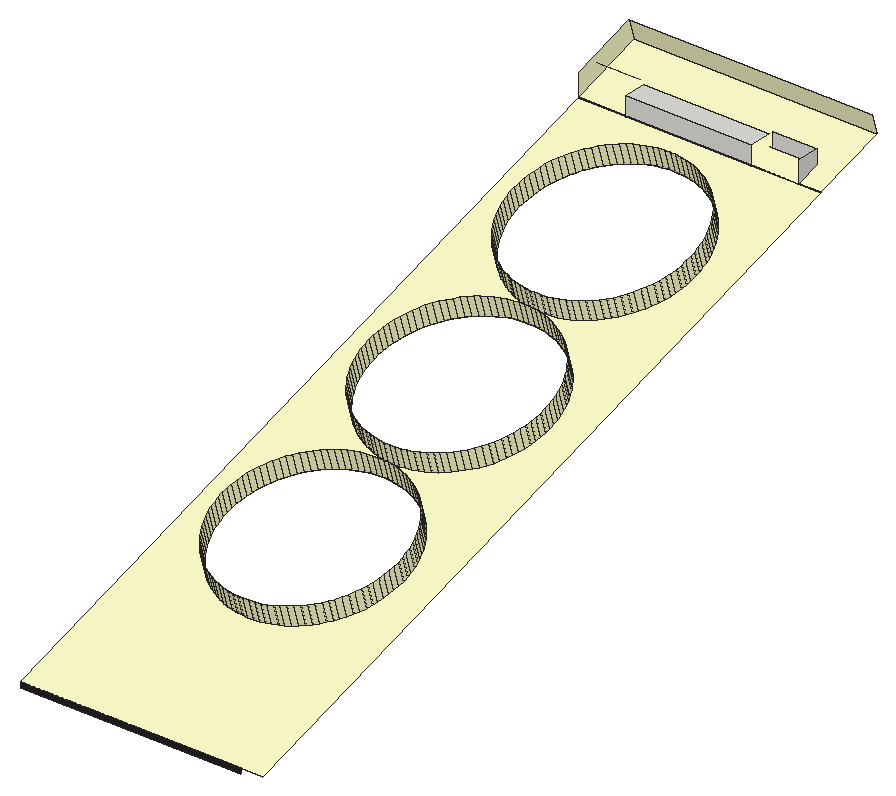
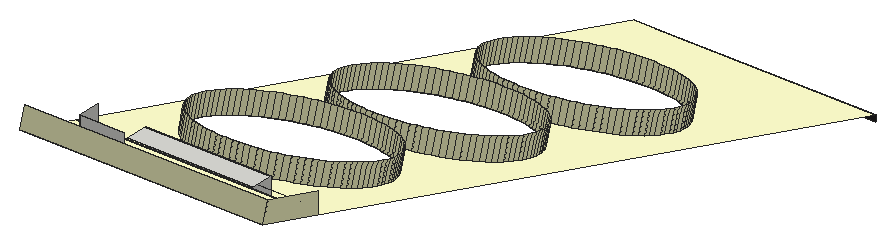
# SketchUp Ruby script. Lengths in inches.
U = 1.inch
M = Sketchup.active_model
def pt(a) = Geom::Point3d.new(a.map { |v| v * U })
def face(e, loops, mat)
  f = e.add_face(loops[0].map { |a| pt(a) })
  loops[1..].each { |l| e.add_face(l.map { |a| pt(a) }).erase! }
  f.material = f.back_material = mat if mat
  f
end
# faces: each face lists its corners as indices into pts; further lists are holes
def faces(e, pts, list, mat = nil) = list.each { |f| face(e, (f[0].is_a?(Array) ? f : [f]).map { |l| l.map { |i| pts[i] } }, mat) }
# xy, xz, yz: faces in a plane at the given z, y or x. An outline is a flat list of corners, or four numbers for a rectangle; further outlines are holes
def ring(l) = l.size == 4 ? [[l[0], l[1]], [l[2], l[1]], [l[2], l[3]], [l[0], l[3]]] : l.each_slice(2).to_a
def flat(e, list, mat, &to3) = list.each { |f| face(e, (f[0].is_a?(Array) ? f : [f]).map { |l| ring(l).map { |u, v| to3.(u, v) } }, mat) }
def xy(e, z, list, mat = nil) = flat(e, list, mat) { |x, y| [x, y, z] }
def xz(e, y, list, mat = nil) = flat(e, list, mat) { |x, z| [x, y, z] }
def yz(e, x, list, mat = nil) = flat(e, list, mat) { |y, z| [x, y, z] }
def lines(e, pts, list) = list.each { |a, b| e.add_line(pt(pts[a]), pt(pts[b])) }
# prism: a flat outline (further loops are holes) pulled along v
def prism(e, loops, v, mat = nil)
  f = face(e, loops, mat); d = Geom::Vector3d.new(v.map { |x| x * U })
  f.pushpull(f.normal.samedirection?(d) ? d.length : -d.length)
end
def box(e, o, s, mat = nil) = prism(e, [[o, [o[0] + s[0], o[1], o[2]], [o[0] + s[0], o[1] + s[1], o[2]], [o[0], o[1] + s[1], o[2]]]], [0, 0, s[2]], mat)
def at(x, y, z, deg = 0) = Geom::Transformation.translation(pt([x, y, z])) * Geom::Transformation.rotation(ORIGIN, Z_AXIS, deg.degrees)
def axes(o, x, y, z) = Geom::Transformation.new([*x, 0, *y, 0, *z, 0, *pt(o).to_a, 1])
def part(name) = M.definitions.add(name)
# library, detail: a bought-in or finely detailed component or shape, given as its bounding box
def library(name, o, s) = part(name).tap { |d| box(d.entities, o, s) }
def detail(e, o, s) = box(e.add_group.entities, o, s)
def put(e, d, t, mat = nil) = e.add_instance(d, t).tap { |i| i.material = mat if mat }
def group(e, t, mat = nil) = e.add_group.tap { |g| g.transformation = t; g.material = mat if mat }.entities
root = M.entities
M.materials.add("E01_Mint_Frost").color = [255, 255, 204]
M.materials.add("Marble_07_1K").color = [36, 34, 36]
xy(root,503,[[276.5,247,310.5,253]])
xz(root,57,[[263.5,437.47,323.5,439.04]],"Marble_07_1K")
xz(root,247,[[263.5,498,276.5,498.15],[276.5,498,310.5,498.15],[310.5,498,323.5,498.15],[323.5,498,329.5,498.15],[276.5,498.15,310.5,503]])
xz(root,253,[[311.5,500.01,323.5,504]])
yz(root,263.5,[[247,498.15,247,504,264.19,509.34,265.85,504,253,500.01]],"E01_Mint_Frost")
yz(root,323.5,[[247,498.15,253,500.01,253,504,247,504]])
p = [[323.5,57,439.04],[263.5,57,439.04],[263.5,247,498],[276.5,247,498],[310.5,247,498],[317.5,247,498],
  [323.5,247,498],[329.5,247,498],[329.5,57,439.04],[273.25,171.72,474.64],[272.93,170.32,474.2],[272.6875,168.89,473.76],
  [272.55,167.46,473.32],[272.5,166.02,472.87],[272.55,164.58,472.42],[272.6875,163.15,471.98],[272.93,161.73,471.54],[273.25,160.32,471.1],
  [273.67,158.9375,470.67],[274.19,157.58,470.25],[274.78,156.26,469.84],[275.47,154.98,469.44],[276.24,153.74,469.06],[277.08,152.55,468.6875],
  [278.01,151.41,468.33],[279,150.33,468],[280.07,149.3125,467.68],[281.2,148.36,467.39],[282.39,147.48,467.11],[283.64,146.67,466.86],
  [284.9375,145.93,466.64],[286.28,145.28,466.43],[287.67,144.71,466.25],[289.08,144.22,466.1],[290.53,143.82,465.98],[292,143.51,465.88],
  [293.49,143.28,465.8125],[294.99,143.14,465.77],[296.5,143.1,465.76],[298.01,143.14,465.77],[299.51,143.28,465.8125],[301,143.51,465.88],
  [302.47,143.82,465.98],[303.92,144.22,466.1],[305.33,144.71,466.25],[306.72,145.28,466.43],[308.0625,145.93,466.64],[309.36,146.67,466.86],
  [310.61,147.48,467.11],[311.8,148.36,467.39],[312.93,149.3125,467.68],[314,150.33,468],[314.99,151.41,468.33],[315.92,152.55,468.6875],
  [316.76,153.74,469.06],[317.53,154.98,469.44],[318.22,156.26,469.84],[318.81,157.58,470.25],[319.33,158.9375,470.67],[319.75,160.32,471.1],
  [320.07,161.73,471.54],[320.3125,163.15,471.98],[320.45,164.58,472.42],[320.5,166.02,472.87],[320.45,167.46,473.32],[320.3125,168.89,473.76],
  [320.07,170.32,474.2],[319.75,171.72,474.64],[319.33,173.1,475.07],[318.81,174.46,475.49],[318.22,175.78,475.9],[317.53,177.0625,476.3],
  [316.76,178.3,476.68],[315.92,179.49,477.05],[314.99,180.63,477.4],[314,181.71,477.74],[312.93,182.73,478.05],[311.8,183.68,478.35],
  [310.61,184.57,478.625],[309.36,185.375,478.875],[308.0625,186.11,479.1],[306.72,186.76,479.31],[305.33,187.33,479.48],[303.92,187.82,479.63],
  [302.47,188.22,479.76],[301,188.54,479.86],[299.51,188.76,479.93],[298.01,188.9,479.97],[296.5,188.94,479.98],[294.99,188.9,479.97],
  [293.49,188.76,479.93],[292,188.54,479.86],[290.53,188.22,479.76],[289.08,187.82,479.63],[287.67,187.33,479.48],[286.28,186.76,479.31],
  [284.9375,186.11,479.1],[283.64,185.375,478.875],[282.39,184.57,478.625],[281.2,183.68,478.35],[280.07,182.73,478.05],[279,181.71,477.74],
  [278.01,180.63,477.4],[277.08,179.49,477.05],[276.24,178.3,476.68],[275.47,177.0625,476.3],[274.78,175.78,475.9],[274.19,174.46,475.49],
  [273.67,173.1,475.07],[272.6875,218.44,489.14],[272.55,217.01,488.69],[272.5,215.57,488.25],[272.55,214.13,487.8],[272.6875,212.7,487.35],
  [272.93,211.28,486.91],[273.25,209.87,486.48],[273.67,208.49,486.05],[274.19,207.13,485.63],[274.78,205.8125,485.22],[275.47,204.53,484.82],
  [276.24,203.29,484.43],[277.08,202.1,484.06],[278.01,200.96,483.71],[279,199.88,483.375],[280.07,198.86,483.0625],[281.2,197.91,482.77],
  [282.39,197.03,482.49],[283.64,196.22,482.24],[284.9375,195.48,482.01],[286.28,194.83,481.81],[287.67,194.26,481.63],[289.08,193.77,481.48],
  [290.53,193.37,481.36],[292,193.06,481.26],[293.49,192.83,481.1875],[294.99,192.69,481.15],[296.5,192.65,481.13],[298.01,192.69,481.15],
  [299.51,192.83,481.1875],[301,193.06,481.26],[302.47,193.37,481.36],[303.92,193.77,481.48],[305.33,194.26,481.63],[306.72,194.83,481.81],
  [308.0625,195.48,482.01],[309.36,196.22,482.24],[310.61,197.03,482.49],[311.8,197.91,482.77],[312.93,198.86,483.0625],[314,199.88,483.375],
  [314.99,200.96,483.71],[315.92,202.1,484.06],[316.76,203.29,484.43],[317.53,204.53,484.82],[318.22,205.8125,485.22],[318.81,207.13,485.63],
  [319.33,208.49,486.05],[319.75,209.87,486.48],[320.07,211.28,486.91],[320.3125,212.7,487.35],[320.45,214.13,487.8],[320.5,215.57,488.25],
  [320.45,217.01,488.69],[320.3125,218.44,489.14],[320.07,219.87,489.58],[319.75,221.27,490.02],[319.33,222.65,490.44],[318.81,224.01,490.86],
  [318.22,225.33,491.27],[317.53,226.61,491.67],[316.76,227.85,492.06],[315.92,229.04,492.43],[314.99,230.18,492.78],[314,231.26,493.12],
  [312.93,232.28,493.43],[311.8,233.23,493.73],[310.61,234.11,494],[309.36,234.92,494.25],[308.0625,235.66,494.48],[306.72,236.3125,494.68],
  [305.33,236.88,494.86],[303.92,237.37,495.01],[302.47,237.77,495.14],[301,238.09,495.23],[299.51,238.3125,495.3],[298.01,238.45,495.35],
  [296.5,238.49,495.36],[294.99,238.45,495.35],[293.49,238.3125,495.3],[292,238.09,495.23],[290.53,237.77,495.14],[289.08,237.37,495.01],
  [287.67,236.88,494.86],[286.28,236.3125,494.68],[284.9375,235.66,494.48],[283.64,234.92,494.25],[282.39,234.11,494],[281.2,233.23,493.73],
  [280.07,232.28,493.43],[279,231.26,493.12],[278.01,230.18,492.78],[277.08,229.04,492.43],[276.24,227.85,492.06],[275.47,226.61,491.67],
  [274.78,225.33,491.27],[274.19,224.01,490.86],[273.67,222.65,490.44],[273.25,221.27,490.02],[272.93,219.87,489.58],[274.19,124.58,460.01],
  [273.67,123.23,459.59],[273.25,121.84,459.16],[272.93,120.4375,458.72],[272.6875,119.02,458.28],[272.55,117.58,457.84],[272.5,116.14,457.39],
  [272.55,114.7,456.94],[272.6875,113.27,456.5],[272.93,111.85,456.06],[273.25,110.44,455.62],[273.67,109.06,455.19],[274.19,107.71,454.77],
  [274.78,106.38,454.36],[275.47,105.1,453.96],[276.24,103.86,453.58],[277.08,102.67,453.21],[278.01,101.53,452.86],[279,100.45,452.52],
  [280.07,99.43,452.2],[281.2,98.48,451.91],[282.39,97.6,451.63],[283.64,96.79,451.38],[284.9375,96.06,451.16],[286.28,95.4,450.95],
  [287.67,94.83,450.78],[289.08,94.34,450.625],[290.53,93.94,450.5],[292,93.63,450.4],[293.49,93.4,450.33],[294.99,93.27,450.29],
  [296.5,93.22,450.28],[298.01,93.27,450.29],[299.51,93.4,450.33],[301,93.63,450.4],[302.47,93.94,450.5],[303.92,94.34,450.625],
  [305.33,94.83,450.78],[306.72,95.4,450.95],[308.0625,96.06,451.16],[309.36,96.79,451.38],[310.61,97.6,451.63],[311.8,98.48,451.91],
  [312.93,99.43,452.2],[314,100.45,452.52],[314.99,101.53,452.86],[315.92,102.67,453.21],[316.76,103.86,453.58],[317.53,105.1,453.96],
  [318.22,106.38,454.36],[318.81,107.71,454.77],[319.33,109.06,455.19],[319.75,110.44,455.62],[320.07,111.85,456.06],[320.3125,113.27,456.5],
  [320.45,114.7,456.94],[320.5,116.14,457.39],[320.45,117.58,457.84],[320.3125,119.02,458.28],[320.07,120.4375,458.72],[319.75,121.84,459.16],
  [319.33,123.23,459.59],[318.81,124.58,460.01],[318.22,125.9,460.42],[317.53,127.1875,460.82],[316.76,128.43,461.2],[315.92,129.62,461.57],
  [314.99,130.75,461.92],[314,131.83,462.26],[312.93,132.85,462.57],[311.8,133.8,462.87],[310.61,134.6875,463.14],[309.36,135.5,463.4],
  [308.0625,136.23,463.625],[306.72,136.88,463.83],[305.33,137.46,464],[303.92,137.94,464.15],[302.47,138.34,464.28],[301,138.66,464.375],
  [299.51,138.88,464.45],[298.01,139.02,464.49],[296.5,139.06,464.5],[294.99,139.02,464.49],[293.49,138.88,464.45],[292,138.66,464.375],
  [290.53,138.34,464.28],[289.08,137.94,464.15],[287.67,137.46,464],[286.28,136.88,463.83],[284.9375,136.23,463.625],[283.64,135.5,463.4],
  [282.39,134.6875,463.14],[281.2,133.8,462.87],[280.07,132.85,462.57],[279,131.83,462.26],[278.01,130.75,461.92],[277.08,129.62,461.57],
  [276.24,128.43,461.2],[275.47,127.1875,460.82],[274.78,125.9,460.42],[294.99,91.57,455.76],[295.01,91.57,455.76],[296.5,91.52,455.75],
  [297.99,91.57,455.76],[298.01,91.57,455.76],[293.49,91.7,455.8],[299.51,91.7,455.8],[292,91.93,455.875],[301,91.93,455.875],
  [290.53,92.24,455.97],[302.47,92.24,455.97],[289.08,92.65,456.1],[303.92,92.65,456.1],[287.67,93.13,456.25],[305.33,93.13,456.25],
  [286.28,93.7,456.43],[306.72,93.7,456.43],[284.9375,94.36,456.63],[308.0625,94.36,456.63],[283.64,95.09,456.86],[309.36,95.09,456.86],
  [282.39,95.9,457.11],[310.61,95.9,457.11],[281.2,96.78,457.38],[311.8,96.78,457.38],[280.07,97.74,457.68],[312.93,97.74,457.68],
  [279,98.75,457.99],[314,98.75,457.99],[278.01,99.83,458.33],[314.99,99.83,458.33],[277.08,100.97,458.68],[315.92,100.97,458.68],
  [276.24,102.16,459.05],[316.76,102.16,459.05],[275.47,103.4,459.44],[317.53,103.4,459.44],[274.78,104.69,459.83],[318.22,104.69,459.83],
  [274.19,106.01,460.24],[318.81,106.01,460.24],[273.67,107.36,460.66],[319.33,107.36,460.66],[273.25,108.74,461.09],[319.75,108.74,461.09],
  [272.93,110.15,461.53],[320.07,110.15,461.53],[272.6875,111.57,461.97],[320.3125,111.57,461.97],[272.55,113.01,462.42],[320.45,113.01,462.42],
  [272.5,114.44,462.86],[320.5,114.44,462.86],[272.55,115.88,463.31],[320.45,115.88,463.31],[272.6875,117.32,463.75],[320.3125,117.32,463.75],
  [272.93,118.74,464.2],[320.07,118.74,464.2],[273.25,120.15,464.63],[319.75,120.15,464.63],[273.67,121.53,465.06],[319.33,121.53,465.06],
  [274.19,122.88,465.48],[318.81,122.88,465.48],[274.78,124.2,465.89],[318.22,124.2,465.89],[275.47,125.49,466.29],[317.53,125.49,466.29],
  [276.24,126.73,466.67],[316.76,126.73,466.67],[277.08,127.92,467.04],[315.92,127.92,467.04],[278.01,129.06,467.4],[314.99,129.06,467.4],
  [279,130.14,467.73],[314,130.14,467.73],[280.07,131.15,468.05],[312.93,131.15,468.05],[281.2,132.11,468.34],[311.8,132.11,468.34],
  [282.39,132.99,468.62],[310.61,132.99,468.62],[283.64,133.8,468.87],[309.36,133.8,468.87],[284.9375,134.53,469.1],[308.0625,134.53,469.1],
  [286.28,135.18,469.3],[306.72,135.18,469.3],[287.67,135.76,469.48],[305.33,135.76,469.48],[289.08,136.24,469.63],[303.92,136.24,469.63],
  [290.53,136.65,469.75],[302.47,136.65,469.75],[292,136.96,469.85],[301,136.96,469.85],[293.49,137.1875,469.92],[299.51,137.1875,469.92],
  [294.99,137.32,469.96],[298.01,137.32,469.96],[296.5,137.37,469.98],[293.49,141.58,471.28],[294.99,141.45,471.24],[296.5,141.4,471.23],
  [298.01,141.45,471.24],[299.51,141.58,471.28],[292,141.81,471.35],[301,141.81,471.35],[290.53,142.12,471.45],[302.47,142.12,471.45],
  [289.08,142.52,471.58],[303.92,142.52,471.58],[287.67,143.01,471.73],[305.33,143.01,471.73],[286.28,143.58,471.91],[306.72,143.58,471.91],
  [284.9375,144.24,472.11],[308.0625,144.24,472.11],[283.64,144.97,472.34],[309.36,144.97,472.34],[282.39,145.78,472.59],[310.61,145.78,472.59],
  [281.2,146.66,472.86],[311.8,146.66,472.86],[280.07,147.61,473.16],[312.93,147.61,473.16],[279,148.63,473.47],[314,148.63,473.47],
  [278.01,149.71,473.81],[314.99,149.71,473.81],[277.08,150.85,474.16],[315.92,150.85,474.16],[276.24,152.04,474.53],[316.76,152.04,474.53],
  [275.47,153.28,474.91],[317.53,153.28,474.91],[274.78,154.5625,475.3125],[318.22,154.5625,475.3125],[274.19,155.88,475.72],[318.81,155.88,475.72],
  [273.67,157.24,476.14],[319.33,157.24,476.14],[273.25,158.62,476.57],[319.75,158.62,476.57],[272.93,160.03,477.01],[320.07,160.03,477.01],
  [272.6875,161.45,477.45],[320.3125,161.45,477.45],[272.55,162.88,477.89],[320.45,162.88,477.89],[272.5,164.32,478.34],[320.5,164.32,478.34],
  [272.55,165.76,478.79],[320.45,165.76,478.79],[272.6875,167.2,479.23],[320.3125,167.2,479.23],[272.93,168.62,479.67],[320.07,168.62,479.67],
  [273.25,170.02,480.11],[319.75,170.02,480.11],[273.67,171.41,480.54],[319.33,171.41,480.54],[274.19,172.76,480.96],[318.81,172.76,480.96],
  [274.78,174.08,481.37],[318.22,174.08,481.37],[275.47,175.37,481.77],[317.53,175.37,481.77],[276.24,176.6,482.15],[316.76,176.6,482.15],
  [277.08,177.8,482.52],[315.92,177.8,482.52],[278.01,178.93,482.875],[314.99,178.93,482.875],[279,180.01,483.21],[314,180.01,483.21],
  [280.07,181.03,483.53],[312.93,181.03,483.53],[281.2,181.98,483.82],[311.8,181.98,483.82],[282.39,182.87,484.1],[310.61,182.87,484.1],
  [283.64,183.68,484.35],[309.36,183.68,484.35],[284.9375,184.41,484.58],[308.0625,184.41,484.58],[286.28,185.0625,484.78],[306.72,185.0625,484.78],
  [287.67,185.63,484.96],[305.33,185.63,484.96],[289.08,186.12,485.11],[303.92,186.12,485.11],[290.53,186.52,485.23],[302.47,186.52,485.23],
  [292,186.84,485.33],[301,186.84,485.33],[293.49,187.0625,485.4],[299.51,187.0625,485.4],[294.99,187.2,485.44],[298.01,187.2,485.44],
  [296.5,187.24,485.46],[295.05,187.2,485.44],[297.95,187.2,485.44],[293.49,191.13,486.66],[294.99,191,486.62],[296.15,190.96,486.61],
  [296.5,190.95,486.61],[296.85,190.96,486.61],[298.01,191,486.62],[299.51,191.13,486.66],[292,191.36,486.73],[301,191.36,486.73],
  [290.53,191.67,486.83],[302.47,191.67,486.83],[289.08,192.07,486.95],[303.92,192.07,486.95],[287.67,192.56,487.1],[305.33,192.56,487.1],
  [286.28,193.13,487.28],[306.72,193.13,487.28],[284.9375,193.79,487.49],[308.0625,193.79,487.49],[283.64,194.52,487.71],[309.36,194.52,487.71],
  [282.39,195.33,487.96],[310.61,195.33,487.96],[281.2,196.21,488.24],[311.8,196.21,488.24],[280.07,197.16,488.53],[312.93,197.16,488.53],
  [279,198.18,488.85],[314,198.18,488.85],[278.01,199.26,489.18],[314.99,199.26,489.18],[277.08,200.4,489.54],[315.92,200.4,489.54],
  [276.24,201.59,489.91],[316.76,201.59,489.91],[275.47,202.83,490.29],[317.53,202.83,490.29],[274.78,204.11,490.69],[318.22,204.11,490.69],
  [274.19,205.43,491.1],[318.81,205.43,491.1],[273.67,206.79,491.52],[319.33,206.79,491.52],[273.25,208.17,491.95],[319.75,208.17,491.95],
  [272.93,209.58,492.39],[320.07,209.58,492.39],[272.6875,211,492.83],[320.3125,211,492.83],[272.55,212.43,493.27],[320.45,212.43,493.27],
  [272.5,213.87,493.72],[320.5,213.87,493.72],[272.55,215.3125,494.17],[320.45,215.3125,494.17],[272.6875,216.74,494.61],[320.3125,216.74,494.61],
  [272.93,218.17,495.05],[320.07,218.17,495.05],[273.25,219.57,495.49],[319.75,219.57,495.49],[273.67,220.96,495.92],[319.33,220.96,495.92],
  [274.19,222.31,496.34],[318.81,222.31,496.34],[274.78,223.63,496.75],[318.22,223.63,496.75],[275.47,224.91,497.15],[317.53,224.91,497.15],
  [276.24,226.15,497.53],[316.76,226.15,497.53],[277.08,227.35,497.9],[315.92,227.35,497.9],[278.01,228.48,498.25],[314.99,228.48,498.25],
  [279,229.5625,498.59],[314,229.5625,498.59],[280.07,230.58,498.9],[312.93,230.58,498.9],[281.2,231.53,499.2],[311.8,231.53,499.2],
  [282.39,232.42,499.47],[310.61,232.42,499.47],[283.64,233.23,499.73],[309.36,233.23,499.73],[284.9375,233.96,499.95],[308.0625,233.96,499.95],
  [286.28,234.61,500.16],[306.72,234.61,500.16],[287.67,235.18,500.33],[305.33,235.18,500.33],[289.08,235.67,500.48],[303.92,235.67,500.48],
  [290.53,236.07,500.61],[302.47,236.07,500.61],[292,236.39,500.71],[301,236.39,500.71],[293.49,236.61,500.78],[299.51,236.61,500.78],
  [294.99,236.75,500.82],[298.01,236.75,500.82],[296.5,236.79,500.83],[296.15,236.78,500.83],[296.85,236.78,500.83],[329.5,265.85,504],
  [329.5,247,498.15],[323.5,247,498.15],[310.5,247,498.15],[276.5,247,498.15],[263.5,247,498.15],[263.5,253,500.01],
  [263.5,265.85,504],[263.5,264.19,509.34],[329.5,264.19,509.34],[275.5,253,504],[263.5,253,504],[310.67,253,500.01],
  [311.5,253,500.01]]
faces(root,p,[[[0,1,2,3,4,5,6,7,8],[9,10,11,12,13,14,15,16,17,18,19,20,21,22,23,24,25,26,27,28,29,30,31,32,33,34,35,36,37,38,39,40,41,42,43,44,45,46,47,48,49,50,51,52,53,54,55,56,57,58,59,60,61,62,63,64,65,66,67,68,69,70,71,72,73,74,75,76,77,78,79,80,81,82,83,84,85,86,87,88,89,90,91,92,93,94,95,96,97,98,99,100,101,102,103,104,105,106,107,108],[109,110,111,112,113,114,115,116,117,118,119,120,121,122,123,124,125,126,127,128,129,130,131,132,133,134,135,136,137,138,139,140,141,142,143,144,145,146,147,148,149,150,151,152,153,154,155,156,157,158,159,160,161,162,163,164,165,166,167,168,169,170,171,172,173,174,175,176,177,178,179,180,181,182,183,184,185,186,187,188,189,190,191,192,193,194,195,196,197,198,199,200,201,202,203,204,205,206,207,208],[209,210,211,212,213,214,215,216,217,218,219,220,221,222,223,224,225,226,227,228,229,230,231,232,233,234,235,236,237,238,239,240,241,242,243,244,245,246,247,248,249,250,251,252,253,254,255,256,257,258,259,260,261,262,263,264,265,266,267,268,269,270,271,272,273,274,275,276,277,278,279,280,281,282,283,284,285,286,287,288,289,290,291,292,293,294,295,296,297,298,299,300,301,302,303,304,305,306,307,308]],[240,239,309,310,311],[241,240,311,312,313],[239,238,314,309],[242,241,313,315],[238,237,316,314],[243,242,315,317],[237,236,318,316],
  [244,243,317,319],[236,235,320,318],[245,244,319,321],[235,234,322,320],[246,245,321,323],[234,233,324,322],[247,246,323,325],[233,232,326,324],
  [248,247,325,327],[232,231,328,326],[249,248,327,329],[231,230,330,328],[250,249,329,331],[230,229,332,330],[251,250,331,333],[229,228,334,332],
  [252,251,333,335],[228,227,336,334],[253,252,335,337],[227,226,338,336],[254,253,337,339],[226,225,340,338],[255,254,339,341],[225,224,342,340],
  [256,255,341,343],[224,223,344,342],[257,256,343,345],[223,222,346,344],[258,257,345,347],[222,221,348,346],[259,258,347,349],[221,220,350,348],
  [260,259,349,351],[220,219,352,350],[261,260,351,353],[219,218,354,352],[262,261,353,355],[218,217,356,354],[263,262,355,357],[217,216,358,356],
  [264,263,357,359],[216,215,360,358],[265,264,359,361],[215,214,362,360],[266,265,361,363],[214,213,364,362],[267,266,363,365],[213,212,366,364],
  [268,267,365,367],[212,211,368,366],[269,268,367,369],[211,210,370,368],[270,269,369,371],[210,209,372,370],[271,270,371,373],[209,308,374,372],
  [272,271,373,375],[308,307,376,374],[273,272,375,377],[307,306,378,376],[274,273,377,379],[306,305,380,378],[275,274,379,381],[305,304,382,380],
  [276,275,381,383],[304,303,384,382],[277,276,383,385],[303,302,386,384],[278,277,385,387],[302,301,388,386],[279,278,387,389],[301,300,390,388],
  [280,279,389,391],[300,299,392,390],[281,280,391,393],[299,298,394,392],[282,281,393,395],[298,297,396,394],[283,282,395,397],[297,296,398,396],
  [284,283,397,399],[296,295,400,398],[285,284,399,401],[295,294,402,400],[286,285,401,403],[294,293,404,402],[287,286,403,405],[293,292,406,404],
  [288,287,405,407],[292,291,408,406],[289,288,407,409],[291,290,410,408],[290,289,409,410],[37,36,411,412],[38,37,412,413],[39,38,413,414],
  [40,39,414,415],[36,35,416,411],[41,40,415,417],[35,34,418,416],[42,41,417,419],[34,33,420,418],[43,42,419,421],[33,32,422,420],
  [44,43,421,423],[32,31,424,422],[45,44,423,425],[31,30,426,424],[46,45,425,427],[30,29,428,426],[47,46,427,429],[29,28,430,428],
  [48,47,429,431],[28,27,432,430],[49,48,431,433],[27,26,434,432],[50,49,433,435],[26,25,436,434],[51,50,435,437],[25,24,438,436],
  [52,51,437,439],[24,23,440,438],[53,52,439,441],[23,22,442,440],[54,53,441,443],[22,21,444,442],[55,54,443,445],[21,20,446,444],
  [56,55,445,447],[20,19,448,446],[57,56,447,449],[19,18,450,448],[58,57,449,451],[18,17,452,450],[59,58,451,453],[17,16,454,452],
  [60,59,453,455],[16,15,456,454],[61,60,455,457],[15,14,458,456],[62,61,457,459],[14,13,460,458],[63,62,459,461],[13,12,462,460],
  [64,63,461,463],[12,11,464,462],[65,64,463,465],[11,10,466,464],[66,65,465,467],[10,9,468,466],[67,66,467,469],[9,108,470,468],
  [68,67,469,471],[108,107,472,470],[69,68,471,473],[107,106,474,472],[70,69,473,475],[106,105,476,474],[71,70,475,477],[105,104,478,476],
  [72,71,477,479],[104,103,480,478],[73,72,479,481],[103,102,482,480],[74,73,481,483],[102,101,484,482],[75,74,483,485],[101,100,486,484],
  [76,75,485,487],[100,99,488,486],[77,76,487,489],[99,98,490,488],[78,77,489,491],[98,97,492,490],[79,78,491,493],[97,96,494,492],
  [80,79,493,495],[96,95,496,494],[81,80,495,497],[95,94,498,496],[82,81,497,499],[94,93,500,498],[83,82,499,501],[93,92,502,500],
  [84,83,501,503],[92,91,504,502],[85,84,503,505],[91,90,506,504],[86,85,505,507],[90,89,508,506],[87,86,507,509],[89,88,510,511,508],
  [88,87,509,512,510],[135,134,513,514],[136,135,514,515,516],[137,136,516,517,518],[138,137,518,519],[134,133,520,513],[139,138,519,521],[133,132,522,520],
  [140,139,521,523],[132,131,524,522],[141,140,523,525],[131,130,526,524],[142,141,525,527],[130,129,528,526],[143,142,527,529],[129,128,530,528],
  [144,143,529,531],[128,127,532,530],[145,144,531,533],[127,126,534,532],[146,145,533,535],[126,125,536,534],[147,146,535,537],[125,124,538,536],
  [148,147,537,539],[124,123,540,538],[149,148,539,541],[123,122,542,540],[150,149,541,543],[122,121,544,542],[151,150,543,545],[121,120,546,544],
  [152,151,545,547],[120,119,548,546],[153,152,547,549],[119,118,550,548],[154,153,549,551],[118,117,552,550],[155,154,551,553],[117,116,554,552],
  [156,155,553,555],[116,115,556,554],[157,156,555,557],[115,114,558,556],[158,157,557,559],[114,113,560,558],[159,158,559,561],[113,112,562,560],
  [160,159,561,563],[112,111,564,562],[161,160,563,565],[111,110,566,564],[162,161,565,567],[110,109,568,566],[163,162,567,569],[109,208,570,568],
  [164,163,569,571],[208,207,572,570],[165,164,571,573],[207,206,574,572],[166,165,573,575],[206,205,576,574],[167,166,575,577],[205,204,578,576],
  [168,167,577,579],[204,203,580,578],[169,168,579,581],[203,202,582,580],[170,169,581,583],[202,201,584,582],[171,170,583,585],[201,200,586,584],
  [172,171,585,587],[200,199,588,586],[173,172,587,589],[199,198,590,588],[174,173,589,591],[198,197,592,590],[175,174,591,593],[197,196,594,592],
  [176,175,593,595],[196,195,596,594],[177,176,595,597],[195,194,598,596],[178,177,597,599],[194,193,600,598],[179,178,599,601],[193,192,602,600],
  [180,179,601,603],[192,191,604,602],[181,180,603,605],[191,190,606,604],[182,181,605,607],[190,189,608,606],[183,182,607,609],[189,188,610,608],
  [184,183,609,611],[188,187,612,610],[185,184,611,613],[187,186,614,615,612],[186,185,613,616,614],[617,618,619,620,621,622,623,624],[624,625,626,617]],"E01_Mint_Frost")
lines(root,p,[[627,628],[629,630]])
